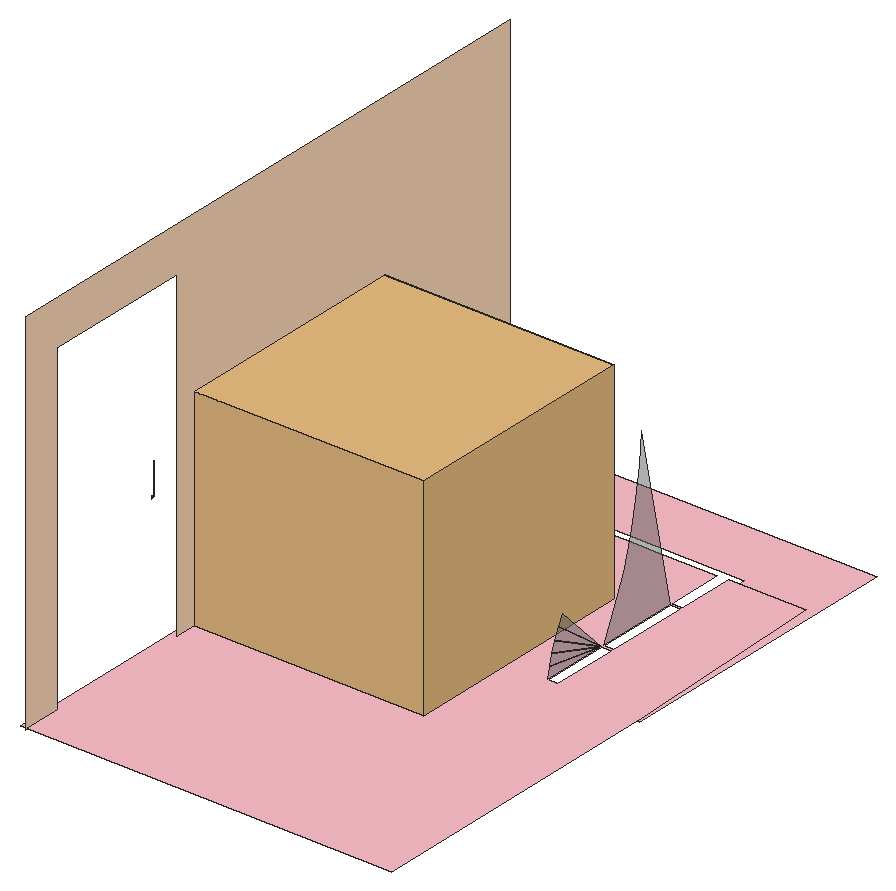
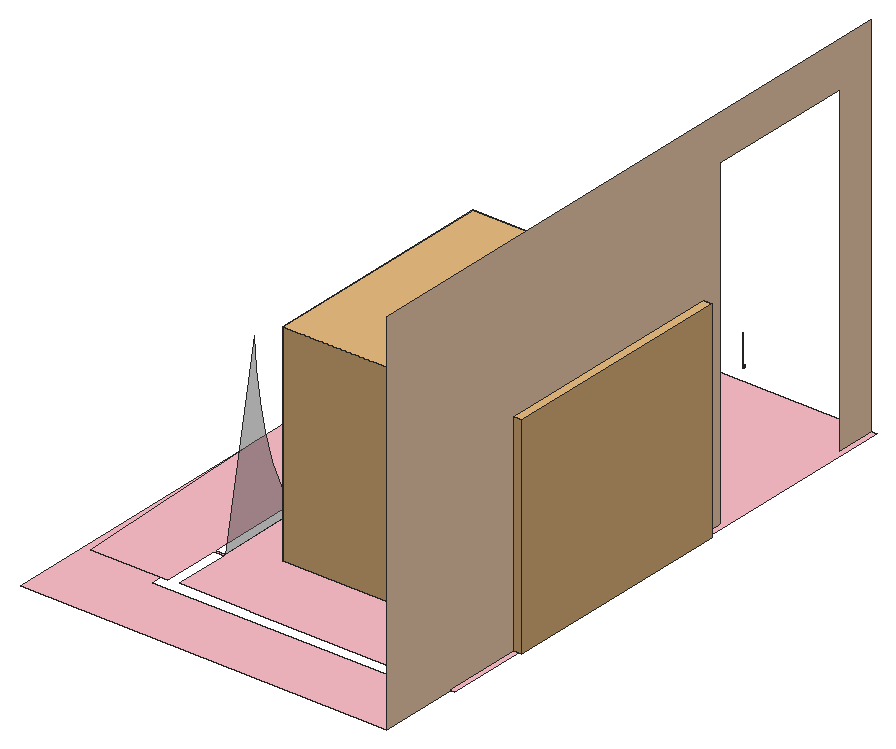
# SketchUp Ruby script. Lengths in inches.
U = 1.inch
M = Sketchup.active_model
def pt(a) = Geom::Point3d.new(a.map { |v| v * U })
def face(e, loops, mat)
  f = e.add_face(loops[0].map { |a| pt(a) })
  loops[1..].each { |l| e.add_face(l.map { |a| pt(a) }).erase! }
  f.material = f.back_material = mat if mat
  f
end
# faces: each face lists its corners as indices into pts; further lists are holes
def faces(e, pts, list, mat = nil) = list.each { |f| face(e, (f[0].is_a?(Array) ? f : [f]).map { |l| l.map { |i| pts[i] } }, mat) }
# xy, xz, yz: faces in a plane at the given z, y or x. An outline is a flat list of corners, or four numbers for a rectangle; further outlines are holes
def ring(l) = l.size == 4 ? [[l[0], l[1]], [l[2], l[1]], [l[2], l[3]], [l[0], l[3]]] : l.each_slice(2).to_a
def flat(e, list, mat, &to3) = list.each { |f| face(e, (f[0].is_a?(Array) ? f : [f]).map { |l| ring(l).map { |u, v| to3.(u, v) } }, mat) }
def xy(e, z, list, mat = nil) = flat(e, list, mat) { |x, y| [x, y, z] }
def xz(e, y, list, mat = nil) = flat(e, list, mat) { |x, z| [x, y, z] }
def yz(e, x, list, mat = nil) = flat(e, list, mat) { |y, z| [x, y, z] }
def lines(e, pts, list) = list.each { |a, b| e.add_line(pt(pts[a]), pt(pts[b])) }
# prism: a flat outline (further loops are holes) pulled along v
def prism(e, loops, v, mat = nil)
  f = face(e, loops, mat); d = Geom::Vector3d.new(v.map { |x| x * U })
  f.pushpull(f.normal.samedirection?(d) ? d.length : -d.length)
end
def box(e, o, s, mat = nil) = prism(e, [[o, [o[0] + s[0], o[1], o[2]], [o[0] + s[0], o[1] + s[1], o[2]], [o[0], o[1] + s[1], o[2]]]], [0, 0, s[2]], mat)
def at(x, y, z, deg = 0) = Geom::Transformation.translation(pt([x, y, z])) * Geom::Transformation.rotation(ORIGIN, Z_AXIS, deg.degrees)
def axes(o, x, y, z) = Geom::Transformation.new([*x, 0, *y, 0, *z, 0, *pt(o).to_a, 1])
def part(name) = M.definitions.add(name)
# library, detail: a bought-in or finely detailed component or shape, given as its bounding box
def library(name, o, s) = part(name).tap { |d| box(d.entities, o, s) }
def detail(e, o, s) = box(e.add_group.entities, o, s)
def put(e, d, t, mat = nil) = e.add_instance(d, t).tap { |i| i.material = mat if mat }
def group(e, t, mat = nil) = e.add_group.tap { |g| g.transformation = t; g.material = mat if mat }.entities
root = M.entities
M.materials.add("Material \#1").color = [140, 140, 140]
M.materials.add("[0006_Pink]").color = [255, 192, 203]
M.materials.add("[0027_PeachPuff]").color = [255, 218, 185]
M.materials.add("[0093_AliceBlue]").color = [240, 248, 255]
M.materials.add("[Translucent Glass Gray]").color = [128, 128, 128]
M.materials["[Translucent Glass Gray]"].alpha = 0.5
c1 = library("Stage Bed",[-27.34,-38.88,0],[54.67,82.38,36.99])
xy(root,0,[[459.4375,249.21,459.4375,323.46,364.5625,323.46,364.5625,345.9375,484.5625,345.9375,484.5625,249.21]],"[0006_Pink]")
xy(root,0.5,[[[362.67,147.9375,362.67,320.52,429.42,320.52,429.42,320.15,453.1,320.15,453.1,301.65,456.54,301.65,456.54,320.52,481.67,320.52,484.33,249.21,484.33,147.9375],[453.17,273.46,456.54,301.21],[453.17,250.71,456.54,272.96]]],"[0006_Pink]")
yz(root,362.57,[[201.94,43.53,202.07,43.57,201.9375,43.55],[201.93,43.79,201.97,43.82,201.92,43.8],[201.92,43.8,201.97,43.82,201.96,43.83],[201.97,43.82,202,43.85,201.96,43.83],[201.96,43.83,202,43.85,201.99,43.86],
  [202.39,43.83,202.4,43.83,202.48,43.9375],[202.39,43.83,202.48,43.9375,202.47,43.95],[202,43.85,202.02,43.89,201.99,43.86],[201.99,43.86,202.02,43.89,202.01,43.9],[202.02,43.89,202.04,43.9375,202.01,43.9],
  [202.01,43.9,202.04,43.9375,202.03,43.94],[202.04,43.9375,202.06,43.98,202.03,43.94],[202.48,43.9375,202.54,44.08,202.47,43.95],[202.03,43.94,202.06,43.98,202.04,43.99],[202.06,43.98,202.0625,44.03,202.04,43.99],
  [202.04,43.99,202.0625,44.03,202.05,44.03],[202.05,44.03,202.06,44.09,202.04,44.08],[202.05,44.03,202.0625,44.03,202.06,44.09],[202.04,44.08,202.04,44.14,202.03,44.13],[202.04,44.08,202.06,44.09,202.04,44.14],
  [202.03,44.13,202.02,44.18,202.01,44.17],[202.03,44.13,202.04,44.14,202.02,44.18],[202.01,44.17,202,44.22,201.99,44.21],[202.01,44.17,202.02,44.18,202,44.22],[201.99,44.21,201.97,44.25,201.96,44.24],
  [201.99,44.21,202,44.22,201.97,44.25],[201.96,44.24,201.93,44.28,201.92,44.27],[201.96,44.24,201.97,44.25,201.93,44.28],[201.92,44.27,201.93,44.28,201.89,44.3]],"Material \#1")
yz(root,362.69,[[201.8,43.52,201.8,43.53,201.94,43.53],[201.8,43.53,201.9375,43.55,201.94,43.53],[201.94,43.53,201.9375,43.55,202.07,43.57],[201.9375,43.55,202.07,43.59,202.07,43.57],[202.07,43.57,202.07,43.59,202.2,43.64],
  [202.07,43.59,202.19,43.65,202.2,43.64],[202.2,43.64,202.19,43.65,202.31,43.72],[202.19,43.65,202.3,43.73,202.31,43.72],[202.31,43.72,202.3,43.73,202.4,43.83],[202.3,43.73,202.39,43.83,202.4,43.83],
  [201.8,43.75,201.8,43.76,201.84,43.75],[201.84,43.75,201.8,43.76,201.84,43.77],[201.84,43.75,201.84,43.77,201.89,43.77],[201.84,43.77,201.88,43.78,201.89,43.77],[201.89,43.77,201.88,43.78,201.93,43.79],
  [201.88,43.78,201.92,43.8,201.93,43.79],[201.93,43.79,201.92,43.8,201.97,43.82],[201.92,43.8,201.96,43.83,201.97,43.82],[201.97,43.82,201.96,43.83,202,43.85],[201.96,43.83,201.99,43.86,202,43.85],
  [202.39,43.83,202.47,43.95,202.48,43.9375],[202.39,43.83,202.48,43.9375,202.4,43.83],[202,43.85,201.99,43.86,202.02,43.89],[201.99,43.86,202.01,43.9,202.02,43.89],[202.02,43.89,202.01,43.9,202.04,43.9375],
  [202.01,43.9,202.03,43.94,202.04,43.9375],[202.04,43.9375,202.03,43.94,202.06,43.98],[202.48,43.9375,202.47,43.95,202.54,44.08],[202.03,43.94,202.04,43.99,202.06,43.98],[202.47,43.95,202.53,44.09,202.54,44.08],
  [202.06,43.98,202.04,43.99,202.0625,44.03],[202.04,43.99,202.05,44.03,202.0625,44.03],[202.05,44.03,202.04,44.08,202.06,44.09],[202.05,44.03,202.06,44.09,202.0625,44.03],[202.04,44.08,202.03,44.13,202.04,44.14],
  [202.04,44.08,202.04,44.14,202.06,44.09],[202.54,44.08,202.53,44.09,202.58,44.23],[202.53,44.09,202.5625,44.23,202.58,44.23],[202.03,44.13,202.01,44.17,202.02,44.18],[202.03,44.13,202.02,44.18,202.04,44.14],
  [202.01,44.17,201.99,44.21,202,44.22],[202.01,44.17,202,44.22,202.02,44.18],[201.99,44.21,201.96,44.24,201.97,44.25],[201.99,44.21,201.97,44.25,202,44.22],[202.5625,44.23,202.58,44.39,202.59,44.39],
  [202.5625,44.23,202.59,44.39,202.58,44.23],[201.96,44.24,201.92,44.27,201.93,44.28],[201.96,44.24,201.93,44.28,201.97,44.25],[201.92,44.27,201.88,44.29,201.89,44.3],[201.92,44.27,201.89,44.3,201.93,44.28],
  [201.88,44.29,201.84,44.3,201.84,44.32],[201.88,44.29,201.84,44.32,201.89,44.3],[201.84,44.3,201.8,44.32,201.84,44.32],[202.58,44.39,202.58,54.24,202.59,54.24],[202.58,44.39,202.59,54.24,202.59,44.39]],"Material \#1")
yz(root,364.5625,[[147.9375,0,160.62,0,160.62,106.4375,209.49,106.4375,209.49,0,345.9375,0,345.9375,121.1875,147.9375,121.1875]],"[0027_PeachPuff]")
p = [[453.17,250.71,0.5],[453.39,251.08,4.22],[453.17,272.96,0.5],[453.63,251.74,7.89],[453.87,252.7,11.5],[454.11,253.95,15.01],
  [454.36,255.48,18.42],[454.125,285.72,38.33],[454.375,286.86,48.24],[454.63,287.21,58.22],[453.17,301.21,0.5],[453.17,273.46,0.5],
  [453.4,277.64,9.5625],[453.63,281.09,18.93],[453.88,283.79,28.54]]
faces(root,p,[[0,1,2],[3,2,1],[4,2,3],[5,2,4],[6,2,5],[7,8,9,10,11,12,13,14]],"[Translucent Glass Gray]")
put(root,c1,axes([402.9,255.48,0.49],[0,1.42296,0],[-0.95046,0,0],[0,0,1.85742]),"[0093_AliceBlue]")
